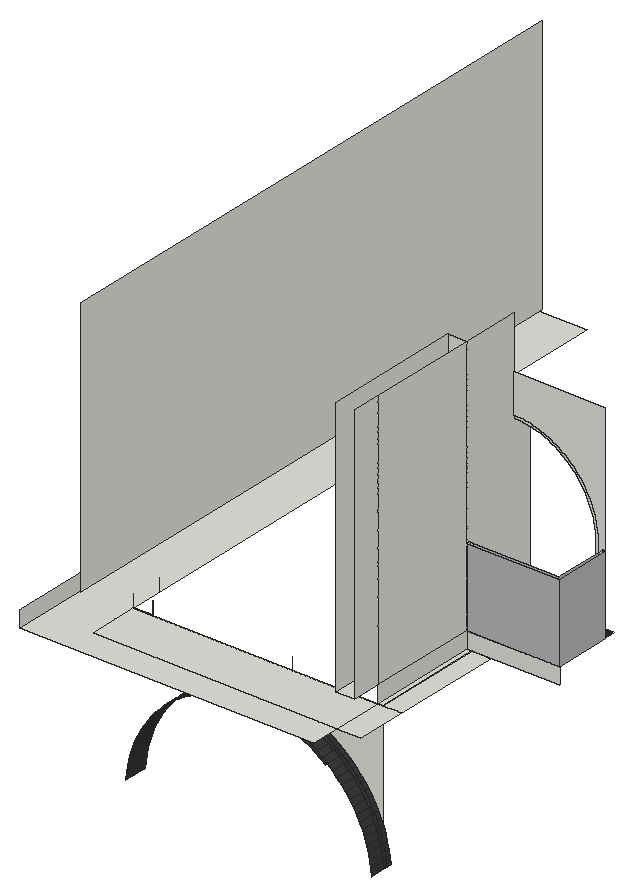
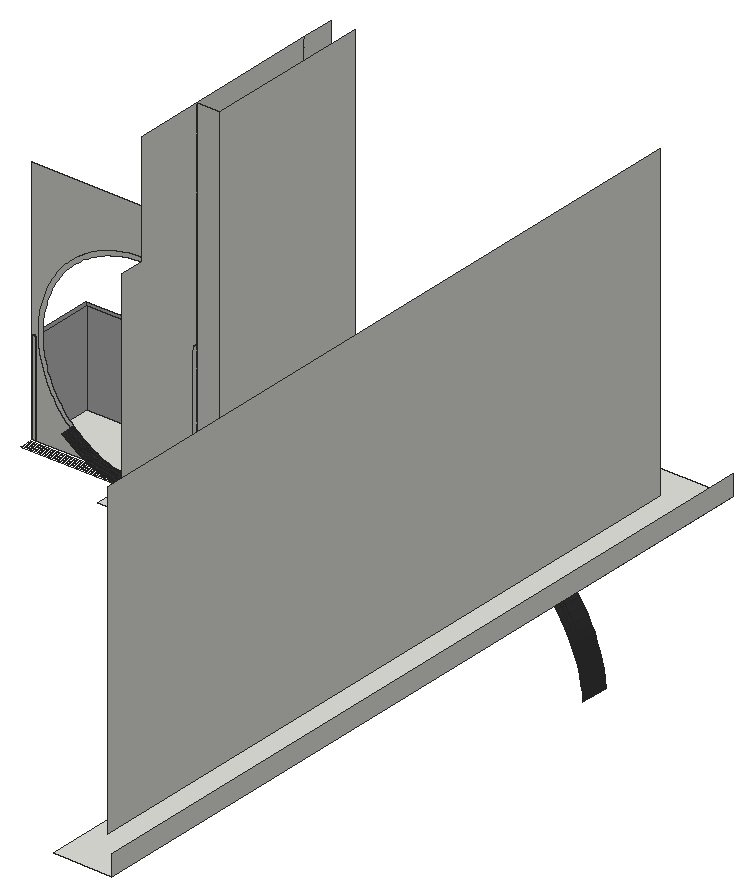
# SketchUp Ruby script. Lengths in inches.
U = 1.inch
M = Sketchup.active_model
def pt(a) = Geom::Point3d.new(a.map { |v| v * U })
def face(e, loops, mat)
  f = e.add_face(loops[0].map { |a| pt(a) })
  loops[1..].each { |l| e.add_face(l.map { |a| pt(a) }).erase! }
  f.material = f.back_material = mat if mat
  f
end
# faces: each face lists its corners as indices into pts; further lists are holes
def faces(e, pts, list, mat = nil) = list.each { |f| face(e, (f[0].is_a?(Array) ? f : [f]).map { |l| l.map { |i| pts[i] } }, mat) }
# xy, xz, yz: faces in a plane at the given z, y or x. An outline is a flat list of corners, or four numbers for a rectangle; further outlines are holes
def ring(l) = l.size == 4 ? [[l[0], l[1]], [l[2], l[1]], [l[2], l[3]], [l[0], l[3]]] : l.each_slice(2).to_a
def flat(e, list, mat, &to3) = list.each { |f| face(e, (f[0].is_a?(Array) ? f : [f]).map { |l| ring(l).map { |u, v| to3.(u, v) } }, mat) }
def xy(e, z, list, mat = nil) = flat(e, list, mat) { |x, y| [x, y, z] }
def xz(e, y, list, mat = nil) = flat(e, list, mat) { |x, z| [x, y, z] }
def yz(e, x, list, mat = nil) = flat(e, list, mat) { |y, z| [x, y, z] }
def lines(e, pts, list) = list.each { |a, b| e.add_line(pt(pts[a]), pt(pts[b])) }
# prism: a flat outline (further loops are holes) pulled along v
def prism(e, loops, v, mat = nil)
  f = face(e, loops, mat); d = Geom::Vector3d.new(v.map { |x| x * U })
  f.pushpull(f.normal.samedirection?(d) ? d.length : -d.length)
end
def box(e, o, s, mat = nil) = prism(e, [[o, [o[0] + s[0], o[1], o[2]], [o[0] + s[0], o[1] + s[1], o[2]], [o[0], o[1] + s[1], o[2]]]], [0, 0, s[2]], mat)
def at(x, y, z, deg = 0) = Geom::Transformation.translation(pt([x, y, z])) * Geom::Transformation.rotation(ORIGIN, Z_AXIS, deg.degrees)
def axes(o, x, y, z) = Geom::Transformation.new([*x, 0, *y, 0, *z, 0, *pt(o).to_a, 1])
def part(name) = M.definitions.add(name)
# library, detail: a bought-in or finely detailed component or shape, given as its bounding box
def library(name, o, s) = part(name).tap { |d| box(d.entities, o, s) }
def detail(e, o, s) = box(e.add_group.entities, o, s)
def put(e, d, t, mat = nil) = e.add_instance(d, t).tap { |i| i.material = mat if mat }
def group(e, t, mat = nil) = e.add_group.tap { |g| g.transformation = t; g.material = mat if mat }.entities
root = M.entities
M.materials.add("[Color M07]").color = [58, 58, 58]
M.materials.add("[Mirror 01]").color = [185, 185, 185]
xy(root,246,[[18.46,0,18.46,299.8125,41.2,299.8125,41.2,37.45,50.2,37.45,50.2,37.13,41.2,37.13,41.2,13.45,154.46,13.45,154.46,0],[41.2,13.45,154.46,37.13],[154.46,13.45,165.63,37.13],[154.46,37.13,156.63,88.96],[156.63,37.13,165.63,88.96],
  [156.63,88.96,165.63,122.64]])
xy(root,253.6875,[[145.46,24,154.46,88.96],[145.46,88.96,154.46,124.96],[154.46,88.96,154.46,90.73,195.57,90.73,195.57,115.33,197.34,115.33,197.34,88.96],[154.46,90.73,156.23,90.73,156.23,113.94,163.81,113.94,163.81,113.57,195.57,113.57,195.57,115.33,165.57,115.33,165.57,115.71,154.46,115.71],[156.23,90.73,195.57,90.73,195.57,113.57,163.81,113.57,163.81,113.94,156.23,113.94],
  [165.57,115.33,175.68,115.71]])
xz(root,37.13,[[156.63,197.34,156.04,198.87,154.78,201.64,153.38,204.34,151.84,206.96,150.16,209.5,148.35,211.94,146.41,214.29,144.35,216.52,142.17,218.65,139.88,220.65,137.49,222.53,135,224.28,132.42,225.9,129.76,227.37,127.02,228.7,124.22,229.89,121.36,230.92,118.45,231.8,115.49,232.52,115,232.61,115,240,156.63,240],[50.2,240,115,246],[115,240,156.63,246]])
xz(root,88.96,[[136.52,246,154.46,253.6875],[154.46,246,197.34,253.6875],[145.46,253.6875,154.46,373.6875]])
xz(root,88.96,[[154.46,253.6875,197.34,289.6875]],"[Mirror 01]")
xz(root,90.73,[[154.46,253.6875,156.23,289.6875]])
xz(root,90.73,[[156.23,253.6875,195.57,289.6875]],"[Mirror 01]")
xz(root,115.33,[[165.57,253.6875,195.57,253.6875,195.57,290.25,197.34,290.25,197.34,349.6875,154.46,349.6875,154.46,331.79,156.04,331.79,156.96,331.75,158.21,331.65,159.46,331.52,160.7,331.34,161.93,331.125,163.16,330.87,164.375,330.58,165.58,330.25,166.78,329.88,167.96,329.47,169.13,329.03,170.29,328.55,171.43,328.04,172.56,327.49,173.66,326.9,174.75,326.28,175.82,325.625,176.87,324.9375,177.89,324.22,178.89,323.46,179.87,322.68,180.82,321.87,181.75,321.03,182.65,320.15,183.52,319.26,184.36,318.33,185.17,317.375,185.96,316.4,186.71,315.4,187.43,314.375,188.12,313.33,188.77,312.26,189.39,311.17,189.98,310.07,190.53,308.94,191.04,307.8,191.52,306.64,191.97,305.47,192.37,304.29,192.74,303.09,193.07,301.88,193.36,300.66,193.62,299.4375,193.83,298.2,194.01,296.96,194.15,295.72,194.24,294.47,194.3,293.22,194.32,291.97,194.3,290.72,194.24,289.47,194.15,288.22,194.01,286.97,193.83,285.73,193.62,284.5,193.36,283.27,193.07,282.06,192.74,280.85,192.37,279.65,191.97,278.47,191.52,277.3,191.04,276.14,190.53,275,189.98,273.87,189.39,272.77,188.77,271.68,188.12,270.61,187.43,269.5625,186.71,268.54,185.96,267.54,185.17,266.5625,184.36,265.61,183.52,264.68,182.65,263.78,181.75,262.91,180.82,262.07,179.87,261.26,178.89,260.47,177.89,259.72,176.87,259,175.82,258.3125,174.75,257.66,173.66,257.04,172.56,256.45,171.43,255.9,170.29,255.39,169.13,254.91,167.96,254.46,166.78,254.06,165.58,253.69],[195.57,253.6875,197.34,289.6875]])
xz(root,115.71,[[156.96,252.1875,158.27,252.29,158.21,252.28],[158.27,252.29,175.68,253.6875,165.57,253.6875,164.375,253.36,163.16,253.07,161.93,252.8125,160.7,252.6,159.46,252.42],[154.46,253.6875,165.57,253.6875,165.58,253.69,166.78,254.06,167.96,254.46,169.13,254.91,170.29,255.39,171.43,255.9,172.56,256.45,173.66,257.04,174.75,257.66,175.82,258.3125,176.87,259,177.89,259.72,178.89,260.47,179.87,261.26,180.82,262.07,181.75,262.91,182.65,263.78,183.52,264.68,184.36,265.61,185.17,266.5625,185.96,267.54,186.71,268.54,187.43,269.5625,188.12,270.61,188.77,271.68,189.39,272.77,189.98,273.87,190.53,275,191.04,276.14,191.52,277.3,191.97,278.47,192.37,279.65,192.74,280.85,193.07,282.06,193.36,283.27,193.62,284.5,193.83,285.73,194.01,286.97,194.15,288.22,194.24,289.47,194.3,290.72,194.32,291.97,194.3,293.22,194.24,294.47,194.15,295.72,194.01,296.96,193.83,298.2,193.62,299.4375,193.36,300.66,193.07,301.88,192.74,303.09,192.37,304.29,191.97,305.47,191.52,306.64,191.04,307.8,190.53,308.94,189.98,310.07,189.39,311.17,188.77,312.26,188.12,313.33,187.43,314.375,186.71,315.4,185.96,316.4,185.17,317.375,184.36,318.33,183.52,319.26,182.65,320.15,181.75,321.03,180.82,321.87,179.87,322.68,178.89,323.46,177.89,324.22,176.87,324.9375,175.82,325.625,174.75,326.28,173.66,326.9,172.56,327.49,171.43,328.04,170.29,328.55,169.13,329.03,167.96,329.47,166.78,329.88,165.58,330.25,164.375,330.58,163.16,330.87,161.93,331.125,160.7,331.34,159.46,331.52,158.21,331.65,156.96,331.75,156.04,331.79,154.46,331.79,154.46,330.25,155.66,330.23,156.86,330.17,158.0625,330.08,159.26,329.95,160.45,329.78,161.63,329.57,162.8125,329.33,163.98,329.05,165.14,328.73,166.29,328.375,167.43,327.99,168.55,327.5625,169.66,327.1,170.76,326.61,171.84,326.08,172.9,325.51,173.95,324.92,174.97,324.29,175.98,323.63,176.96,322.9375,177.92,322.22,178.86,321.46,179.78,320.68,180.67,319.875,181.53,319.04,182.37,318.17,183.18,317.28,183.96,316.37,184.71,315.43,185.43,314.47,186.12,313.49,186.78,312.48,187.41,311.46,188.01,310.41,188.57,309.35,189.1,308.27,189.59,307.17,190.05,306.0625,190.48,304.9375,190.87,303.8,191.22,302.65,191.54,301.49,191.82,300.32,192.0625,299.14,192.27,297.96,192.44,296.77,192.57,295.57,192.67,294.37,192.72,293.17,192.74,291.97,192.72,290.77,192.67,289.57,192.57,288.37,192.44,287.17,192.27,285.98,192.0625,284.8,191.82,283.62,191.54,282.45,191.22,281.29,190.87,280.14,190.48,279,190.05,277.875,189.59,276.77,189.1,275.67,188.57,274.59,188.01,273.53,187.41,272.48,186.78,271.46,186.12,270.45,185.43,269.47,184.71,268.51,183.96,267.57,183.18,266.65,182.37,265.76,181.53,264.9,180.67,264.0625,179.78,263.25,178.86,262.47,177.92,261.72,176.96,261,175.98,260.31,174.97,259.65,173.95,259.02,172.9,258.42,171.84,257.86,170.76,257.33,169.66,256.84,168.55,256.375,167.43,255.95,166.29,255.5625,165.14,255.21,163.98,254.89,162.8125,254.61,161.63,254.37,160.45,254.16,159.26,253.99,158.0625,253.86,156.86,253.76,155.66,253.71]])
yz(root,18.46,[[0,246,299.8125,253.6875]])
yz(root,27.46,[[24,253.6875,290.8125,373.6875]])
yz(root,50.2,[[37.13,240,37.45,246],[37.13,246,37.45,252]])
yz(root,145.46,[[24,253.6875,88.96,373.6875]])
yz(root,154.46,[[37.13,246,88.96,253.6875],[24,253.6875,37.13,373.6875],[37.13,253.6875,88.96,373.6875],[88.96,253.6875,90.73,289.6875],[90.73,253.6875,124.96,253.6875,124.96,330.25,115.71,330.25,115.71,331.79,115.33,331.79,115.33,349.6875,115.71,349.6875,115.71,373.6875,88.96,373.6875,88.96,290.25,90.73,290.25]])
yz(root,156.63,[[37.13,240,122.64,246]])
yz(root,195.57,[[113.57,253.6875,115.33,289.6875]])
yz(root,195.57,[[90.73,253.6875,113.57,289.6875]],"[Mirror 01]")
yz(root,197.34,[[88.96,253.6875,115.33,289.6875]],"[Mirror 01]")
p = [[46.5,26.33,181.21],[46.5,33.16,181.21],[46.82,33.16,184.23],[46.82,26.33,184.23],[160.01,26.33,184.23],[160.01,33.16,184.23],
  [160.33,33.16,181.21],[160.33,26.33,181.21],[46.82,34.78,184.23],[46.5,34.78,181.21],[160.33,34.78,181.21],[160.01,34.78,184.23],
  [46.82,37.13,184.23],[46.5,37.13,181.21],[160.33,37.13,181.21],[160.01,37.13,184.23],[47.3,33.16,187.24],[47.3,26.33,187.24],
  [159.53,26.33,187.24],[159.53,33.16,187.24],[47.3,34.78,187.24],[159.53,34.78,187.24],[47.3,37.13,187.24],[159.53,37.13,187.24],
  [47.9375,33.16,190.21],[47.9375,26.33,190.21],[158.89,26.33,190.21],[158.89,33.16,190.21],[47.9375,34.78,190.21],[158.89,34.78,190.21],
  [47.9375,37.13,190.21],[158.89,37.13,190.21],[48.73,33.16,193.15],[48.73,26.33,193.15],[158.09,26.33,193.15],[158.09,33.16,193.15],
  [48.73,34.78,193.15],[158.09,34.78,193.15],[48.73,37.13,193.15],[158.09,37.13,193.15],[49.6875,33.16,196.03],[49.6875,26.33,196.03],
  [157.14,26.33,196.03],[157.14,33.16,196.03],[49.6875,34.78,196.03],[157.14,34.78,196.03],[49.6875,37.13,196.03],[157.14,37.13,196.03],
  [50.79,33.16,198.87],[50.79,26.33,198.87],[156.04,26.33,198.87],[156.04,33.16,198.87],[50.79,34.78,198.87],[156.04,34.78,198.87],
  [50.79,37.13,198.87],[156.04,37.13,198.87],[156.63,37.13,197.34],[52.05,33.16,201.64],[52.05,26.33,201.64],[154.78,26.33,201.64],
  [154.78,33.16,201.64],[52.05,34.78,201.64],[154.78,34.78,201.64],[52.05,37.13,201.64],[154.78,37.13,201.64],[53.45,33.16,204.34],
  [53.45,26.33,204.34],[153.38,26.33,204.34],[153.38,33.16,204.34],[53.45,34.78,204.34],[153.38,34.78,204.34],[53.45,37.13,204.34],
  [153.38,37.13,204.34],[54.99,33.16,206.96],[54.99,26.33,206.96],[151.84,26.33,206.96],[151.84,33.16,206.96],[54.99,34.78,206.96],
  [151.84,34.78,206.96],[54.99,37.13,206.96],[151.84,37.13,206.96],[56.67,33.16,209.5],[56.67,26.33,209.5],[150.16,26.33,209.5],
  [150.16,33.16,209.5],[56.67,34.78,209.5],[150.16,34.78,209.5],[56.67,37.13,209.5],[150.16,37.13,209.5],[58.48,33.16,211.94],
  [58.48,26.33,211.94],[148.35,26.33,211.94],[148.35,33.16,211.94],[58.48,34.78,211.94],[148.35,34.78,211.94],[58.48,37.13,211.94],
  [148.35,37.13,211.94],[60.42,33.16,214.29],[60.42,26.33,214.29],[146.41,26.33,214.29],[146.41,33.16,214.29],[60.42,34.78,214.29],
  [146.41,34.78,214.29],[60.42,37.13,214.29],[146.41,37.13,214.29],[62.48,33.16,216.52],[62.48,26.33,216.52],[144.35,26.33,216.52],
  [144.35,33.16,216.52],[62.48,34.78,216.52],[144.35,34.78,216.52],[62.48,37.13,216.52],[144.35,37.13,216.52],[64.66,33.16,218.65],
  [64.66,26.33,218.65],[142.17,26.33,218.65],[142.17,33.16,218.65],[64.66,34.78,218.65],[142.17,34.78,218.65],[64.66,37.13,218.65],
  [142.17,37.13,218.65],[64.66,25.27,218.65],[66.95,26.33,220.65],[66.95,25.27,220.65],[66.95,33.16,220.65],[139.88,26.33,220.65],
  [139.88,33.16,220.65],[66.95,34.78,220.65],[139.88,34.78,220.65],[66.95,37.13,220.65],[139.88,37.13,220.65],[69.34,26.33,222.53],
  [69.34,25.27,222.53],[137.49,25.27,222.53],[137.49,26.33,222.53],[139.88,25.27,220.65],[69.34,33.16,222.53],[137.49,32.53,222.53],
  [137.49,33.16,222.53],[69.34,34.78,222.53],[137.49,34.78,222.53],[69.34,37.13,222.53],[137.49,37.13,222.53],[71.83,26.33,224.28],
  [71.83,25.27,224.28],[135,25.27,224.28],[135,26.33,224.28],[69.46,33.16,222.61],[69.46,32.53,222.61],[70.64,32.53,223.45],
  [70.64,33.16,223.45],[71.83,33.16,224.28],[135,33.16,224.28],[136.24,33.16,223.41],[136.24,32.53,223.41],[71.83,34.78,224.28],
  [135,34.78,224.28],[71.83,37.13,224.28],[135,37.13,224.28],[74.41,26.33,225.9],[74.41,25.27,225.9],[132.42,25.27,225.9],
  [132.42,26.33,225.9],[74.41,33.16,225.9],[132.42,33.16,225.9],[74.41,34.78,225.9],[132.42,34.78,225.9],[74.41,37.13,225.9],
  [132.42,37.13,225.9],[77.07,26.33,227.37],[77.07,25.27,227.37],[129.76,25.27,227.37],[129.76,26.33,227.37],[77.07,33.16,227.37],
  [129.76,33.16,227.37],[77.07,34.78,227.37],[129.76,34.78,227.37],[77.07,37.13,227.37],[129.76,37.13,227.37],[79.81,26.33,228.7],
  [79.81,25.27,228.7],[127.02,25.27,228.7],[127.02,26.33,228.7],[79.81,33.16,228.7],[127.02,33.16,228.7],[79.81,34.78,228.7],
  [127.02,34.78,228.7],[79.81,37.13,228.7],[127.02,37.13,228.7],[82.61,26.33,229.89],[82.61,25.27,229.89],[124.22,25.27,229.89],
  [124.22,26.33,229.89],[82.61,33.16,229.89],[124.22,33.16,229.89],[82.61,34.78,229.89],[124.22,34.78,229.89],[82.61,37.13,229.89],
  [124.22,37.13,229.89],[85.47,26.33,230.92],[85.47,25.27,230.92],[121.36,25.27,230.92],[121.36,26.33,230.92],[85.47,33.16,230.92],
  [121.36,33.16,230.92],[85.47,34.78,230.92],[121.36,34.78,230.92],[85.47,37.13,230.92],[121.36,37.13,230.92],[88.38,26.33,231.8],
  [88.38,25.27,231.8],[118.45,25.27,231.8],[118.45,26.33,231.8],[88.38,33.16,231.8],[118.45,33.16,231.8],[88.38,34.78,231.8],
  [118.45,34.78,231.8],[88.38,37.13,231.8],[118.45,37.13,231.8],[91.34,26.33,232.52],[91.34,25.27,232.52],[115.49,25.27,232.52],
  [115.49,26.33,232.52],[91.34,33.16,232.52],[115.49,33.16,232.52],[91.34,34.78,232.52],[115.49,34.78,232.52],[91.34,37.13,232.52],
  [115.49,37.13,232.52],[94.33,26.33,233.08],[94.33,25.27,233.08],[112.5,25.27,233.08],[112.5,26.33,233.08],[94.33,33.16,233.08],
  [112.5,33.16,233.08],[94.33,34.78,233.08],[112.5,34.78,233.08],[94.33,37.13,233.08],[112.5,37.13,233.08],[115,37.13,232.61],
  [97.34,26.33,233.49],[97.34,25.27,233.49],[109.49,25.27,233.49],[109.49,26.33,233.49],[97.34,33.16,233.49],[109.49,33.16,233.49],
  [97.34,34.78,233.49],[109.49,34.78,233.49],[97.34,37.13,233.49],[109.49,37.13,233.49],[100.375,26.33,233.73],[100.375,25.27,233.73],
  [106.46,25.27,233.73],[106.46,26.33,233.73],[100.375,33.16,233.73],[106.46,33.16,233.73],[100.375,34.78,233.73],[106.46,34.78,233.73],
  [100.375,37.13,233.73],[106.46,37.13,233.73],[103.41,26.33,233.8125],[103.41,25.27,233.8125],[101.89,33.16,233.77],[101.89,32.53,233.77],
  [103.41,32.53,233.8125],[103.41,33.16,233.8125],[103.41,34.78,233.8125],[103.41,37.13,233.8125],[165.58,115.71,253.69],[165.57,115.71,253.6875],
  [165.57,115.33,253.6875],[165.58,115.33,253.69],[166.78,115.71,254.06],[166.78,115.33,254.06],[155.66,115.71,253.71],[155.66,116.39,253.71],
  [154.46,116.39,253.6875],[154.46,115.71,253.6875],[156.86,115.71,253.76],[156.86,116.39,253.76],[155.66,117.08,253.71],[154.46,117.08,253.6875],
  [156.86,117.08,253.76],[155.66,117.77,253.71],[154.46,117.77,253.6875],[156.86,117.77,253.76],[155.66,118.46,253.71],[154.46,118.46,253.6875],
  [156.86,118.46,253.76],[155.66,119.14,253.71],[154.46,119.14,253.6875],[156.86,119.14,253.76],[155.66,119.83,253.71],[154.46,119.83,253.6875],
  [156.86,119.83,253.76],[155.66,120.52,253.71],[154.46,120.52,253.6875],[156.86,120.52,253.76],[155.66,121.21,253.71],[154.46,121.21,253.6875],
  [156.86,121.21,253.76],[155.66,121.89,253.71],[154.46,121.89,253.6875],[156.86,121.89,253.76],[158.0625,115.71,253.86],[158.0625,116.39,253.86],
  [158.0625,117.08,253.86],[158.0625,117.77,253.86],[158.0625,118.46,253.86],[158.0625,119.14,253.86],[158.0625,119.83,253.86],[158.0625,120.52,253.86],
  [158.0625,121.21,253.86],[158.0625,121.89,253.86],[159.26,115.71,253.99],[159.26,116.39,253.99],[159.26,117.08,253.99],[159.26,117.77,253.99],
  [159.26,118.46,253.99],[159.26,119.14,253.99],[159.26,119.83,253.99],[159.26,120.52,253.99],[159.26,121.21,253.99],[159.26,121.89,253.99],
  [160.45,115.71,254.16],[160.45,116.39,254.16],[160.45,117.08,254.16],[160.45,117.77,254.16],[160.45,118.46,254.16],[160.45,119.14,254.16],
  [160.45,119.83,254.16],[160.45,120.52,254.16],[160.45,121.21,254.16],[160.45,121.89,254.16],[167.96,115.71,254.46],[167.96,115.33,254.46],
  [161.63,115.71,254.37],[161.63,116.39,254.37],[161.63,117.08,254.37],[161.63,117.77,254.37],[161.63,118.46,254.37],[161.63,119.14,254.37],
  [161.63,119.83,254.37],[161.63,120.52,254.37],[161.63,121.21,254.37],[161.63,121.89,254.37],[162.8125,115.71,254.61],[162.8125,116.39,254.61],
  [162.8125,117.08,254.61],[162.8125,117.77,254.61],[162.8125,118.46,254.61],[162.8125,119.14,254.61],[162.8125,119.83,254.61],[162.8125,120.52,254.61],
  [162.8125,121.21,254.61],[169.13,115.71,254.91],[169.13,115.33,254.91],[163.98,115.71,254.89],[163.98,116.39,254.89],[163.98,117.08,254.89],
  [163.98,117.77,254.89],[163.98,118.46,254.89],[163.98,119.14,254.89],[163.98,119.83,254.89],[163.98,120.52,254.89],[163.98,121.21,254.89],
  [170.29,115.71,255.39],[170.29,115.33,255.39],[165.14,115.71,255.21],[165.14,116.39,255.21],[165.14,117.08,255.21],[165.14,117.77,255.21],
  [165.14,118.46,255.21],[165.14,119.14,255.21],[165.14,119.83,255.21],[165.14,120.52,255.21],[165.14,121.21,255.21],[166.29,115.71,255.5625],
  [166.29,116.39,255.5625],[166.29,117.08,255.5625],[166.29,117.77,255.5625],[166.29,118.46,255.5625],[166.29,119.14,255.5625],[166.29,119.83,255.5625],
  [166.29,120.52,255.5625],[166.29,121.21,255.5625],[171.43,115.71,255.9],[171.43,115.33,255.9],[167.43,115.71,255.95],[167.43,116.39,255.95],
  [167.43,117.08,255.95],[167.43,117.77,255.95],[167.43,118.46,255.95],[167.43,119.14,255.95],[167.43,119.83,255.95],[167.43,120.52,255.95],
  [167.43,121.21,255.95],[172.56,115.71,256.45],[172.56,115.33,256.45],[168.55,115.71,256.375],[168.55,116.39,256.375],[168.55,117.08,256.375],
  [168.55,117.77,256.375],[168.55,118.46,256.375],[168.55,119.14,256.375],[168.55,119.83,256.375],[168.55,120.52,256.375],[168.55,121.21,256.375],
  [169.66,115.71,256.84],[169.66,116.39,256.84],[169.66,117.08,256.84],[169.66,117.77,256.84],[169.66,118.46,256.84],[169.66,119.14,256.84],
  [169.66,119.83,256.84],[169.66,120.52,256.84],[169.66,121.21,256.84],[173.66,115.71,257.04],[173.66,115.33,257.04],[170.76,115.71,257.33],
  [170.76,116.39,257.33],[170.76,117.08,257.33],[170.76,117.77,257.33],[170.76,118.46,257.33],[170.76,119.14,257.33],[170.76,119.83,257.33],
  [170.76,120.52,257.33],[170.76,121.21,257.33],[174.75,115.71,257.66],[174.75,115.33,257.66],[171.84,115.71,257.86],[171.84,116.39,257.86],
  [171.84,117.08,257.86],[171.84,117.77,257.86],[171.84,118.46,257.86],[171.84,119.14,257.86],[171.84,119.83,257.86],[171.84,120.52,257.86],
  [171.84,121.21,257.86],[175.82,115.71,258.3125],[175.82,115.33,258.3125],[172.9,115.71,258.42],[172.9,116.39,258.42],[172.9,117.08,258.42],
  [172.9,117.77,258.42],[172.9,118.46,258.42],[172.9,119.14,258.42],[172.9,119.83,258.42],[172.9,120.52,258.42],[172.9,121.21,258.42],
  [176.87,115.71,259],[176.87,115.33,259],[173.95,115.71,259.02],[173.95,116.39,259.02],[173.95,117.08,259.02],[173.95,117.77,259.02],
  [173.95,118.46,259.02],[173.95,119.14,259.02],[173.95,119.83,259.02],[173.95,120.52,259.02],[173.95,121.21,259.02],[177.89,115.71,259.72],
  [177.89,115.33,259.72],[174.97,115.71,259.65],[174.97,116.39,259.65],[174.97,117.08,259.65],[174.97,117.77,259.65],[174.97,118.46,259.65],
  [174.97,119.14,259.65],[174.97,119.83,259.65],[174.97,120.52,259.65],[174.97,121.21,259.65],[175.98,115.71,260.31],[175.98,116.39,260.31],
  [175.98,117.08,260.31],[175.98,117.77,260.31],[175.98,118.46,260.31],[175.98,119.14,260.31],[175.98,119.83,260.31],[175.98,120.52,260.31],
  [175.98,121.21,260.31],[178.89,115.71,260.47],[178.89,115.33,260.47],[176.96,115.71,261],[176.96,116.39,261],[176.96,117.08,261],
  [176.96,117.77,261],[176.96,118.46,261],[176.96,119.14,261],[176.96,119.83,261],[176.96,120.52,261],[176.96,121.21,261],
  [179.87,115.71,261.26],[179.87,115.33,261.26],[177.92,115.71,261.72],[177.92,116.39,261.72],[177.92,117.08,261.72],[177.92,117.77,261.72],
  [177.92,118.46,261.72],[177.92,119.14,261.72],[177.92,119.83,261.72],[177.92,120.52,261.72],[177.92,121.21,261.72],[180.82,115.71,262.07],
  [180.82,115.33,262.07],[178.86,115.71,262.47],[178.86,116.39,262.47],[178.86,117.08,262.47],[178.86,117.77,262.47],[178.86,118.46,262.47],
  [178.86,119.14,262.47],[178.86,119.83,262.47],[178.86,120.52,262.47],[178.86,121.21,262.47],[181.75,115.71,262.91],[181.75,115.33,262.91],
  [179.78,115.71,263.25],[179.78,116.39,263.25],[179.78,117.08,263.25],[179.78,117.77,263.25],[179.78,118.46,263.25],[179.78,119.14,263.25],
  [179.78,119.83,263.25],[179.78,120.52,263.25],[179.78,121.21,263.25],[182.65,115.71,263.78],[182.65,115.33,263.78],[180.67,115.71,264.0625],
  [180.67,116.39,264.0625],[180.67,117.08,264.0625],[180.67,117.77,264.0625],[180.67,118.46,264.0625],[180.67,119.14,264.0625],[180.67,119.83,264.0625],
  [180.67,120.52,264.0625],[180.67,121.21,264.0625],[41.2,37.13,246],[41.2,37.13,252],[41.2,52.07,246],[41.2,52.07,252],
  [41.2,37.45,246],[41.2,37.45,252],[115,37.13,246],[115,37.13,252],[196.96,116.39,253.6875],[196.96,117.08,253.6875],
  [196.96,117.77,253.6875],[196.96,118.46,253.6875],[196.96,119.14,253.6875],[196.96,119.83,253.6875],[196.96,120.52,253.6875],[196.96,121.21,253.6875]]
faces(root,p,[[0,1,2,3],[4,5,6,7],[8,9,1,2],[10,11,5,6],[12,8,9,13],[14,10,11,15],[3,2,16,17],[18,19,5,4],
  [20,8,2,16],[11,21,19,5],[22,20,8,12],[15,11,21,23],[17,16,24,25],[26,27,19,18],[28,20,16,24],[21,29,27,19],
  [30,28,20,22],[23,21,29,31],[25,24,32,33],[34,35,27,26],[36,28,24,32],[29,37,35,27],[38,36,28,30],[31,29,37,39],
  [33,32,40,41],[42,43,35,34],[44,36,32,40],[37,45,43,35],[46,44,36,38],[39,37,45,47],[41,40,48,49],[50,51,43,42],
  [52,44,40,48],[45,53,51,43],[54,52,44,46],[47,45,53,55,56],[49,48,57,58],[59,60,51,50],[61,52,48,57],[53,62,60,51],
  [63,61,52,54],[55,53,62,64],[58,57,65,66],[67,68,60,59],[69,61,57,65],[62,70,68,60],[71,69,61,63],[64,62,70,72],
  [66,65,73,74],[75,76,68,67],[77,69,65,73],[70,78,76,68],[79,77,69,71],[72,70,78,80],[74,73,81,82],[83,84,76,75],
  [85,77,73,81],[78,86,84,76],[87,85,77,79],[80,78,86,88],[82,81,89,90],[91,92,84,83],[93,85,81,89],[86,94,92,84],
  [95,93,85,87],[88,86,94,96],[90,89,97,98],[99,100,92,91],[101,93,89,97],[94,102,100,92],[103,101,93,95],[96,94,102,104],
  [98,97,105,106],[107,108,100,99],[109,101,97,105],[102,110,108,100],[111,109,101,103],[104,102,110,112],[106,105,113,114],[115,116,108,107],
  [117,109,105,113],[110,118,116,108],[119,117,109,111],[112,110,118,120],[121,114,122,123],[114,113,124,122],[125,126,116,115],[127,117,113,124],
  [118,128,126,116],[129,127,117,119],[120,118,128,130],[123,122,131,132],[133,134,125,135],[122,124,136,131],[137,138,126,125,134],[139,127,124,136],
  [128,140,138,126],[141,139,127,129],[130,128,140,142],[132,131,143,144],[145,146,134,133],[131,136,147,148,149,150,151,143],[146,152,153,154,137,134],[153,138,137,154],
  [139,155,151,150,147,136],[140,156,152,153,138],[157,155,139,141],[142,140,156,158],[150,147,148,149],[144,143,159,160],[161,162,146,145],[143,151,163,159],
  [162,164,152,146],[165,155,151,163],[156,166,164,152],[167,165,155,157],[158,156,166,168],[160,159,169,170],[171,172,162,161],[159,163,173,169],
  [172,174,164,162],[175,165,163,173],[166,176,174,164],[177,175,165,167],[168,166,176,178],[170,169,179,180],[181,182,172,171],[169,173,183,179],
  [182,184,174,172],[185,175,173,183],[176,186,184,174],[187,185,175,177],[178,176,186,188],[180,179,189,190],[191,192,182,181],[179,183,193,189],
  [192,194,184,182],[195,185,183,193],[186,196,194,184],[197,195,185,187],[188,186,196,198],[190,189,199,200],[201,202,192,191],[189,193,203,199],
  [202,204,194,192],[205,195,193,203],[196,206,204,194],[207,205,195,197],[198,196,206,208],[200,199,209,210],[211,212,202,201],[199,203,213,209],
  [212,214,204,202],[215,205,203,213],[206,216,214,204],[217,215,205,207],[208,206,216,218],[210,209,219,220],[221,222,212,211],[209,213,223,219],
  [222,224,214,212],[225,215,213,223],[216,226,224,214],[227,225,215,217],[218,216,226,228],[220,219,229,230],[231,232,222,221],[219,223,233,229],
  [232,234,224,222],[235,225,223,233],[226,236,234,224],[237,235,225,227],[228,226,236,238,239],[230,229,240,241],[242,243,232,231],[229,233,244,240],
  [243,245,234,232],[246,235,233,244],[236,247,245,234],[248,246,235,237],[238,236,247,249],[241,240,250,251],[252,253,243,242],[240,244,254,250],
  [253,255,245,243],[256,246,244,254],[247,257,255,245],[258,256,246,248],[249,247,257,259],[251,250,260,261],[261,260,253,252],[250,254,262,263,264,260],
  [264,265,255,253,260],[266,256,254,262,265],[257,266,265,255],[267,266,256,258],[259,257,266,267],[262,265,264,263],[274,275,276,277],[278,279,275,274],
  [275,280,281,276],[279,282,280,275],[280,283,284,281],[282,285,283,280],[283,286,287,284],[285,288,286,283],[286,289,290,287],[288,291,289,286],
  [289,292,293,290],[291,294,292,289],[292,295,296,293],[294,297,295,292],[295,298,299,296],[297,300,298,295],[298,301,302,299],[300,303,301,298],
  [304,305,279,278],[305,306,282,279],[306,307,285,282],[307,308,288,285],[308,309,291,288],[309,310,294,291],[310,311,297,294],[311,312,300,297],
  [312,313,303,300],[314,315,305,304],[315,316,306,305],[316,317,307,306],[317,318,308,307],[318,319,309,308],[319,320,310,309],[320,321,311,310],
  [321,322,312,311],[322,323,313,312],[324,325,315,314],[325,326,316,315],[326,327,317,316],[327,328,318,317],[328,329,319,318],[329,330,320,319],
  [330,331,321,320],[331,332,322,321],[332,333,323,322],[336,337,325,324],[337,338,326,325],[338,339,327,326],[339,340,328,327],[340,341,329,328],
  [341,342,330,329],[342,343,331,330],[343,344,332,331],[344,345,333,332],[346,347,337,336],[347,348,338,337],[348,349,339,338],[349,350,340,339],
  [350,351,341,340],[351,352,342,341],[352,353,343,342],[353,354,344,343],[357,358,347,346],[358,359,348,347],[359,360,349,348],[360,361,350,349],
  [361,362,351,350],[362,363,352,351],[363,364,353,352],[364,365,354,353],[368,369,358,357],[369,370,359,358],[370,371,360,359],[371,372,361,360],
  [372,373,362,361],[373,374,363,362],[374,375,364,363],[375,376,365,364],[377,378,369,368],[378,379,370,369],[379,380,371,370],[380,381,372,371],
  [381,382,373,372],[382,383,374,373],[383,384,375,374],[384,385,376,375],[388,389,378,377],[389,390,379,378],[390,391,380,379],[391,392,381,380],
  [392,393,382,381],[393,394,383,382],[394,395,384,383],[395,396,385,384],[399,400,389,388],[400,401,390,389],[401,402,391,390],[402,403,392,391],
  [403,404,393,392],[404,405,394,393],[405,406,395,394],[406,407,396,395],[408,409,400,399],[409,410,401,400],[410,411,402,401],[411,412,403,402],
  [412,413,404,403],[413,414,405,404],[414,415,406,405],[415,416,407,406],[419,420,409,408],[420,421,410,409],[421,422,411,410],[422,423,412,411],
  [423,424,413,412],[424,425,414,413],[425,426,415,414],[426,427,416,415],[430,431,420,419],[431,432,421,420],[432,433,422,421],[433,434,423,422],
  [434,435,424,423],[435,436,425,424],[436,437,426,425],[437,438,427,426],[441,442,431,430],[442,443,432,431],[443,444,433,432],[444,445,434,433],
  [445,446,435,434],[446,447,436,435],[447,448,437,436],[448,449,438,437],[452,453,442,441],[453,454,443,442],[454,455,444,443],[455,456,445,444],
  [456,457,446,445],[457,458,447,446],[458,459,448,447],[459,460,449,448],[463,464,453,452],[464,465,454,453],[465,466,455,454],[466,467,456,455],
  [467,468,457,456],[468,469,458,457],[469,470,459,458],[470,471,460,459],[472,473,464,463],[473,474,465,464],[474,475,466,465],[475,476,467,466],
  [476,477,468,467],[477,478,469,468],[478,479,470,469],[479,480,471,470],[483,484,473,472],[484,485,474,473],[485,486,475,474],[486,487,476,475],
  [487,488,477,476],[488,489,478,477],[489,490,479,478],[490,491,480,479],[494,495,484,483],[495,496,485,484],[496,497,486,485],[497,498,487,486],
  [498,499,488,487],[499,500,489,488],[500,501,490,489],[501,502,491,490],[505,506,495,494],[506,507,496,495],[507,508,497,496],[508,509,498,497],
  [509,510,499,498],[510,511,500,499],[511,512,501,500],[512,513,502,501],[516,517,506,505],[517,518,507,506],[518,519,508,507],[519,520,509,508],
  [520,521,510,509],[521,522,511,510],[522,523,512,511],[523,524,513,512],[527,528,517,516],[528,529,518,517],[529,530,519,518],[530,531,520,519],
  [531,532,521,520],[532,533,522,521],[533,534,523,522],[534,535,524,523]],"[Color M07]")
faces(root,p,[[268,269,270,271],[272,268,271,273],[334,272,273,335],[355,334,335,356],[366,355,356,367],[386,366,367,387],[397,386,387,398],[417,397,398,418],
  [428,417,418,429],[439,428,429,440],[450,439,440,451],[461,450,451,462],[481,461,462,482],[492,481,482,493],[503,492,493,504],[514,503,504,515],
  [525,514,515,526]])
lines(root,p,[[536,537],[538,539],[540,541],[542,543],[544,276],[545,281],[546,284],[547,287],[548,290],[549,293],[550,296],[551,299]])
